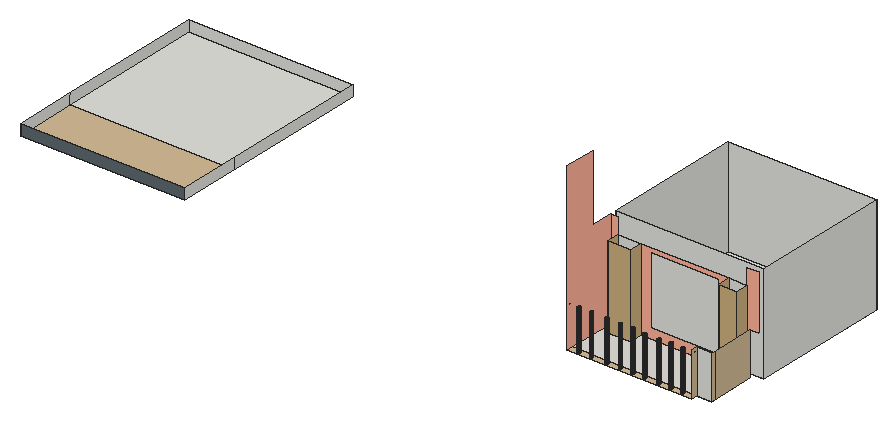
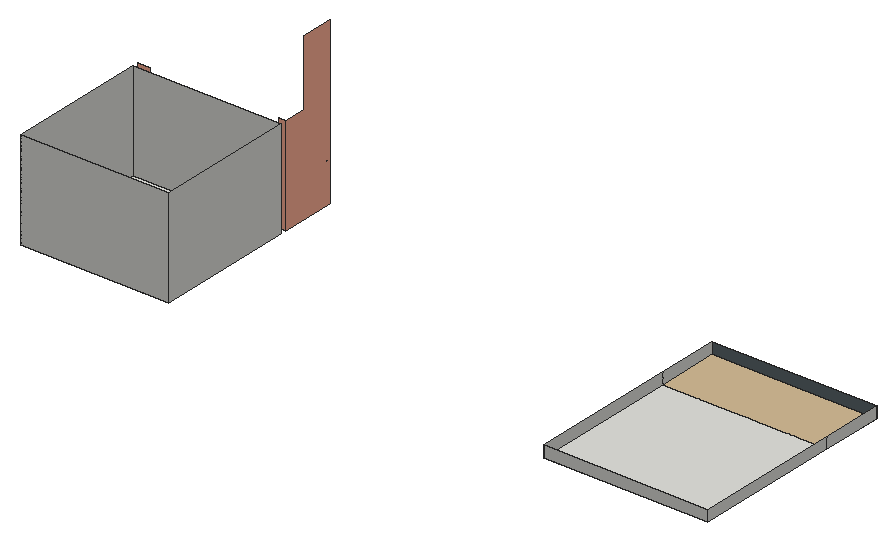
# SketchUp Ruby script. Lengths in inches.
U = 1.inch
M = Sketchup.active_model
def pt(a) = Geom::Point3d.new(a.map { |v| v * U })
def face(e, loops, mat)
  f = e.add_face(loops[0].map { |a| pt(a) })
  loops[1..].each { |l| e.add_face(l.map { |a| pt(a) }).erase! }
  f.material = f.back_material = mat if mat
  f
end
# faces: each face lists its corners as indices into pts; further lists are holes
def faces(e, pts, list, mat = nil) = list.each { |f| face(e, (f[0].is_a?(Array) ? f : [f]).map { |l| l.map { |i| pts[i] } }, mat) }
# xy, xz, yz: faces in a plane at the given z, y or x. An outline is a flat list of corners, or four numbers for a rectangle; further outlines are holes
def ring(l) = l.size == 4 ? [[l[0], l[1]], [l[2], l[1]], [l[2], l[3]], [l[0], l[3]]] : l.each_slice(2).to_a
def flat(e, list, mat, &to3) = list.each { |f| face(e, (f[0].is_a?(Array) ? f : [f]).map { |l| ring(l).map { |u, v| to3.(u, v) } }, mat) }
def xy(e, z, list, mat = nil) = flat(e, list, mat) { |x, y| [x, y, z] }
def xz(e, y, list, mat = nil) = flat(e, list, mat) { |x, z| [x, y, z] }
def yz(e, x, list, mat = nil) = flat(e, list, mat) { |y, z| [x, y, z] }
def lines(e, pts, list) = list.each { |a, b| e.add_line(pt(pts[a]), pt(pts[b])) }
# prism: a flat outline (further loops are holes) pulled along v
def prism(e, loops, v, mat = nil)
  f = face(e, loops, mat); d = Geom::Vector3d.new(v.map { |x| x * U })
  f.pushpull(f.normal.samedirection?(d) ? d.length : -d.length)
end
def box(e, o, s, mat = nil) = prism(e, [[o, [o[0] + s[0], o[1], o[2]], [o[0] + s[0], o[1] + s[1], o[2]], [o[0], o[1] + s[1], o[2]]]], [0, 0, s[2]], mat)
def at(x, y, z, deg = 0) = Geom::Transformation.translation(pt([x, y, z])) * Geom::Transformation.rotation(ORIGIN, Z_AXIS, deg.degrees)
def axes(o, x, y, z) = Geom::Transformation.new([*x, 0, *y, 0, *z, 0, *pt(o).to_a, 1])
def part(name) = M.definitions.add(name)
# library, detail: a bought-in or finely detailed component or shape, given as its bounding box
def library(name, o, s) = part(name).tap { |d| box(d.entities, o, s) }
def detail(e, o, s) = box(e.add_group.entities, o, s)
def put(e, d, t, mat = nil) = e.add_instance(d, t).tap { |i| i.material = mat if mat }
def group(e, t, mat = nil) = e.add_group.tap { |g| g.transformation = t; g.material = mat if mat }.entities
root = M.entities
M.materials.add("[Color B02]").color = [255, 178, 153]
M.materials.add("[Formica Beige]").color = [211, 187, 149]
M.materials.add("[Formica Laminate Dark]").color = [50, 53, 60]
M.materials.add("[Formica Speckled Grey]").color = [94, 105, 111]
M.materials.add("[Terrazzo Tile Accent]").color = [224, 221, 217]
M.materials.add("[Wood Floor Light]").color = [204, 176, 127]
xy(root,501,[[621.3,124.73,620.89,124.78,620.51,124.94,620.19,125.1875,619.94,125.51,619.79,125.89,619.73,126.29,619.79,126.7,619.94,127.07,620.19,127.4,620.51,127.65,620.89,127.8,621.3,127.86,621.7,127.8,622.08,127.65,622.4,127.4,622.65,127.07,622.81,126.7,622.86,126.29,622.81,125.89,622.65,125.51,622.4,125.1875,622.08,124.94,621.7,124.78],[634.92,124.73,634.52,124.78,634.14,124.94,633.82,125.1875,633.57,125.51,633.41,125.89,633.36,126.29,633.41,126.7,633.57,127.07,633.82,127.4,634.14,127.65,634.52,127.8,634.92,127.86,635.33,127.8,635.7,127.65,636.03,127.4,636.27,127.07,636.43,126.7,636.48,126.29,636.43,125.89,636.27,125.51,636.03,125.1875,635.7,124.94,635.33,124.78],[651.73,124.73,651.33,124.78,650.95,124.94,650.63,125.1875,650.38,125.51,650.22,125.89,650.17,126.29,650.22,126.7,650.38,127.07,650.63,127.4,650.95,127.65,651.33,127.8,651.73,127.86,652.14,127.8,652.51,127.65,652.84,127.4,653.09,127.07,653.24,126.7,653.3,126.29,653.24,125.89,653.09,125.51,652.84,125.1875,652.51,124.94,652.14,124.78],[666.73,124.73,666.33,124.78,665.95,124.94,665.63,125.1875,665.38,125.51,665.22,125.89,665.17,126.29,665.22,126.7,665.38,127.07,665.63,127.4,665.95,127.65,666.33,127.8,666.73,127.86,667.14,127.8,667.51,127.65,667.84,127.4,668.09,127.07,668.24,126.7,668.3,126.29,668.24,125.89,668.09,125.51,667.84,125.1875,667.51,124.94,667.14,124.78],[680.8,124.73,680.39,124.78,680.01,124.94,679.69,125.1875,679.44,125.51,679.29,125.89,679.23,126.29,679.29,126.7,679.44,127.07,679.69,127.4,680.01,127.65,680.39,127.8,680.8,127.86,681.2,127.8,681.58,127.65,681.9,127.4,682.15,127.07,682.31,126.7,682.36,126.29,682.31,125.89,682.15,125.51,681.9,125.1875,681.58,124.94,681.2,124.78],
  [693.42,124.73,693.02,124.78,692.64,124.94,692.32,125.1875,692.07,125.51,691.91,125.89,691.86,126.29,691.91,126.7,692.07,127.07,692.32,127.4,692.64,127.65,693.02,127.8,693.42,127.86,693.83,127.8,694.2,127.65,694.53,127.4,694.77,127.07,694.93,126.7,694.98,126.29,694.93,125.89,694.77,125.51,694.53,125.1875,694.2,124.94,693.83,124.78],[709.48,124.73,709.08,124.78,708.7,124.94,708.38,125.1875,708.13,125.51,707.97,125.89,707.92,126.29,707.97,126.7,708.13,127.07,708.38,127.4,708.7,127.65,709.08,127.8,709.48,127.86,709.89,127.8,710.26,127.65,710.59,127.4,710.84,127.07,710.99,126.7,711.05,126.29,710.99,125.89,710.84,125.51,710.59,125.1875,710.26,124.94,709.89,124.78],[722.42,124.73,722.02,124.78,721.64,124.94,721.32,125.1875,721.07,125.51,720.91,125.89,720.86,126.29,720.91,126.7,721.07,127.07,721.32,127.4,721.64,127.65,722.02,127.8,722.42,127.86,722.83,127.8,723.2,127.65,723.53,127.4,723.77,127.07,723.93,126.7,723.98,126.29,723.93,125.89,723.77,125.51,723.53,125.1875,723.2,124.94,722.83,124.78],[735.61,124.73,735.2,124.78,734.83,124.94,734.5,125.1875,734.26,125.51,734.1,125.89,734.05,126.29,734.1,126.7,734.26,127.07,734.5,127.4,734.83,127.65,735.2,127.8,735.61,127.86,736.01,127.8,736.39,127.65,736.71,127.4,736.96,127.07,737.12,126.7,737.17,126.29,737.12,125.89,736.96,125.51,736.71,125.1875,736.39,124.94,736.01,124.78],[619.29,168.64,644.11,182.57],
  [741.11,168.64,761.42,182.57],[611.125,189.24,774.15,344.36],[9,191.15,189.57,355.125]])
xy(root,501,[[9,122.79,189.57,191.15],[[611.125,122.79,748.22,130.07],[621.3,124.73,620.89,124.78,620.51,124.94,620.19,125.1875,619.94,125.51,619.79,125.89,619.73,126.29,619.79,126.7,619.94,127.07,620.19,127.4,620.51,127.65,620.89,127.8,621.3,127.86,621.7,127.8,622.08,127.65,622.4,127.4,622.65,127.07,622.81,126.7,622.86,126.29,622.81,125.89,622.65,125.51,622.4,125.1875,622.08,124.94,621.7,124.78],[722.42,124.73,722.02,124.78,721.64,124.94,721.32,125.1875,721.07,125.51,720.91,125.89,720.86,126.29,720.91,126.7,721.07,127.07,721.32,127.4,721.64,127.65,722.02,127.8,722.42,127.86,722.83,127.8,723.2,127.65,723.53,127.4,723.77,127.07,723.93,126.7,723.98,126.29,723.93,125.89,723.77,125.51,723.53,125.1875,723.2,124.94,722.83,124.78],[634.92,124.73,634.52,124.78,634.14,124.94,633.82,125.1875,633.57,125.51,633.41,125.89,633.36,126.29,633.41,126.7,633.57,127.07,633.82,127.4,634.14,127.65,634.52,127.8,634.92,127.86,635.33,127.8,635.7,127.65,636.03,127.4,636.27,127.07,636.43,126.7,636.48,126.29,636.43,125.89,636.27,125.51,636.03,125.1875,635.7,124.94,635.33,124.78],[709.48,124.73,709.08,124.78,708.7,124.94,708.38,125.1875,708.13,125.51,707.97,125.89,707.92,126.29,707.97,126.7,708.13,127.07,708.38,127.4,708.7,127.65,709.08,127.8,709.48,127.86,709.89,127.8,710.26,127.65,710.59,127.4,710.84,127.07,710.99,126.7,711.05,126.29,710.99,125.89,710.84,125.51,710.59,125.1875,710.26,124.94,709.89,124.78],[651.73,124.73,651.33,124.78,650.95,124.94,650.63,125.1875,650.38,125.51,650.22,125.89,650.17,126.29,650.22,126.7,650.38,127.07,650.63,127.4,650.95,127.65,651.33,127.8,651.73,127.86,652.14,127.8,652.51,127.65,652.84,127.4,653.09,127.07,653.24,126.7,653.3,126.29,653.24,125.89,653.09,125.51,652.84,125.1875,652.51,124.94,652.14,124.78],[693.42,124.73,693.02,124.78,692.64,124.94,692.32,125.1875,692.07,125.51,691.91,125.89,691.86,126.29,691.91,126.7,692.07,127.07,692.32,127.4,692.64,127.65,693.02,127.8,693.42,127.86,693.83,127.8,694.2,127.65,694.53,127.4,694.77,127.07,694.93,126.7,694.98,126.29,694.93,125.89,694.77,125.51,694.53,125.1875,694.2,124.94,693.83,124.78],[666.73,124.73,666.33,124.78,665.95,124.94,665.63,125.1875,665.38,125.51,665.22,125.89,665.17,126.29,665.22,126.7,665.38,127.07,665.63,127.4,665.95,127.65,666.33,127.8,666.73,127.86,667.14,127.8,667.51,127.65,667.84,127.4,668.09,127.07,668.24,126.7,668.3,126.29,668.24,125.89,668.09,125.51,667.84,125.1875,667.51,124.94,667.14,124.78],[680.8,124.73,680.39,124.78,680.01,124.94,679.69,125.1875,679.44,125.51,679.29,125.89,679.23,126.29,679.29,126.7,679.44,127.07,679.69,127.4,680.01,127.65,680.39,127.8,680.8,127.86,681.2,127.8,681.58,127.65,681.9,127.4,682.15,127.07,682.31,126.7,682.36,126.29,682.31,125.89,682.15,125.51,681.9,125.1875,681.58,124.94,681.2,124.78],[735.61,124.73,735.2,124.78,734.83,124.94,734.5,125.1875,734.26,125.51,734.1,125.89,734.05,126.29,734.1,126.7,734.26,127.07,734.5,127.4,734.83,127.65,735.2,127.8,735.61,127.86,736.01,127.8,736.39,127.65,736.71,127.4,736.96,127.07,737.12,126.7,737.17,126.29,737.12,125.89,736.96,125.51,736.71,125.1875,736.39,124.94,736.01,124.78]]],"[Formica Beige]")
xy(root,501,[[611.125,130.07,764.59,130.07,764.59,182.57,761.42,182.57,761.42,168.64,741.11,168.64,741.11,182.57,644.11,182.57,644.11,168.64,619.29,168.64,619.29,182.57,611.125,182.57]],"[Terrazzo Tile Accent]")
xz(root,122.79,[[9,501,189.57,513]],"[Formica Speckled Grey]")
xz(root,130.07,[[748.22,501,764.59,549]])
xz(root,168.64,[[619.29,501,644.11,591.38],[741.11,501,761.42,591.38]],"[Wood Floor Light]")
xz(root,182.57,[[619.29,501,644.11,591.38],[741.11,501,761.42,591.38]])
xz(root,182.57,[[611.125,501,619.29,609],[[644.11,501,741.11,591.38],[654.83,511.625,730.21,587]],[761.42,501,764.59,501,764.59,549,774.15,549,774.15,609,761.42,609]],"[Color B02]")
xz(root,189.24,[[611.125,501,774.15,609]])
xz(root,344.36,[[611.125,501,774.15,609]])
xz(root,355.125,[[9,501,189.57,513]])
yz(root,9,[[122.79,501,191.15,513],[191.15,501,355.125,513]])
yz(root,189.57,[[122.79,501,191.15,513],[191.15,501,355.125,513]])
yz(root,611.125,[[189.24,501,344.36,609]])
yz(root,611.125,[[[122.79,501,182.57,501,182.57,609,157.7,609,157.7,682.5,122.79,682.5],[126.51,543.63,126.14,543.68,125.79,543.82,125.49,544.05,125.26,544.35,125.12,544.69,125.07,545.07,125.12,545.4375,125.26,545.78,125.49,546.08,125.79,546.31,126.14,546.45,126.51,546.5,126.88,546.45,127.23,546.31,127.52,546.08,127.75,545.78,127.9,545.4375,127.95,545.07,127.9,544.69,127.75,544.35,127.52,544.05,127.23,543.82,126.88,543.68]]],"[Color B02]")
yz(root,619.29,[[168.64,501,182.57,591.38]],"[Wood Floor Light]")
yz(root,644.11,[[168.64,501,182.57,591.38]],"[Wood Floor Light]")
yz(root,741.11,[[168.64,501,182.57,591.38]],"[Wood Floor Light]")
yz(root,748.22,[[[122.79,501,130.07,549],[126.51,543.63,126.88,543.68,127.23,543.82,127.52,544.05,127.75,544.35,127.9,544.69,127.95,545.07,127.9,545.4375,127.75,545.78,127.52,546.08,127.23,546.31,126.88,546.45,126.51,546.5,126.14,546.45,125.79,546.31,125.49,546.08,125.26,545.78,125.12,545.4375,125.07,545.07,125.12,544.69,125.26,544.35,125.49,544.05,125.79,543.82,126.14,543.68]]],"[Formica Beige]")
yz(root,761.42,[[168.64,501,182.57,591.38]],"[Wood Floor Light]")
yz(root,764.59,[[130.07,501,133.51,549],[133.51,501,182.57,549]],"[Formica Beige]")
yz(root,774.15,[[189.24,501,344.36,609]])
p = [[620.89,124.78,501],[621.3,124.73,501],[621.3,124.73,545.4375],[620.89,124.78,545.4375],[621.7,124.78,501],[621.7,124.78,545.4375],
  [634.52,124.78,501],[634.92,124.73,501],[634.92,124.73,545.4375],[634.52,124.78,545.4375],[635.33,124.78,501],[635.33,124.78,545.4375],
  [651.33,124.78,501],[651.73,124.73,501],[651.73,124.73,545.4375],[651.33,124.78,545.4375],[652.14,124.78,501],[652.14,124.78,545.4375],
  [666.33,124.78,501],[666.73,124.73,501],[666.73,124.73,544.8125],[666.33,124.78,544.8125],[667.14,124.78,501],[667.14,124.78,544.8125],
  [680.39,124.78,501],[680.8,124.73,501],[680.8,124.73,545.78],[680.39,124.78,545.78],[681.2,124.78,501],[681.2,124.78,545.78],
  [693.02,124.78,501],[693.42,124.73,501],[693.42,124.73,544.8125],[693.02,124.78,544.8125],[693.83,124.78,501],[693.83,124.78,544.8125],
  [709.08,124.78,501],[709.48,124.73,501],[709.48,124.73,544.8125],[709.08,124.78,544.8125],[709.89,124.78,501],[709.89,124.78,544.8125],
  [722.02,124.78,501],[722.42,124.73,501],[722.42,124.73,545.78],[722.02,124.78,545.78],[722.83,124.78,501],[722.83,124.78,545.78],
  [735.2,124.78,501],[735.61,124.73,501],[735.61,124.73,545.4375],[735.2,124.78,545.4375],[736.01,124.78,501],[736.01,124.78,545.4375],
  [620.51,124.94,501],[620.51,124.94,545.4375],[622.08,124.94,501],[622.08,124.94,545.4375],[634.14,124.94,501],[634.14,124.94,545.4375],
  [635.7,124.94,501],[635.7,124.94,545.4375],[650.95,124.94,501],[650.95,124.94,545.4375],[652.51,124.94,501],[652.51,124.94,545.4375],
  [665.95,124.94,501],[665.95,124.94,544.8125],[667.51,124.94,501],[667.51,124.94,544.8125],[680.01,124.94,501],[680.01,124.94,545.78],
  [681.58,124.94,501],[681.58,124.94,545.78],[692.64,124.94,501],[692.64,124.94,544.8125],[694.2,124.94,501],[694.2,124.94,544.8125],
  [708.7,124.94,501],[708.7,124.94,544.8125],[710.26,124.94,501],[710.26,124.94,544.8125],[721.64,124.94,501],[721.64,124.94,545.78],
  [723.2,124.94,501],[723.2,124.94,545.78],[734.83,124.94,501],[734.83,124.94,545.4375],[736.39,124.94,501],[736.39,124.94,545.4375],
  [620.19,125.1875,501],[620.28,125.12,545.4375],[620.19,125.1875,545.4375],[622.4,125.1875,501],[622.4,125.1875,545.4375],[622.3125,125.12,545.4375],
  [633.82,125.1875,501],[633.91,125.12,545.4375],[633.82,125.1875,545.4375],[636.03,125.1875,501],[636.03,125.1875,545.4375],[635.9375,125.12,545.4375],
  [650.63,125.1875,501],[650.72,125.12,545.4375],[650.63,125.1875,545.4375],[652.84,125.1875,501],[652.84,125.1875,545.4375],[652.75,125.12,545.4375],
  [665.63,125.1875,501],[665.63,125.1875,544.8125],[667.84,125.1875,501],[667.84,125.1875,544.8125],[679.69,125.1875,501],[679.69,125.1875,545.78],
  [681.9,125.1875,501],[681.9,125.1875,545.78],[692.32,125.1875,501],[692.32,125.1875,544.8125],[694.53,125.1875,501],[694.53,125.1875,544.8125],
  [708.38,125.1875,501],[708.38,125.1875,544.8125],[710.59,125.1875,501],[710.59,125.1875,544.8125],[721.32,125.1875,501],[721.32,125.1875,545.78],
  [723.53,125.1875,501],[723.53,125.1875,545.78],[734.5,125.1875,501],[734.59,125.12,545.4375],[734.5,125.1875,545.4375],[736.71,125.1875,501],
  [736.71,125.1875,545.4375],[736.625,125.12,545.4375],[619.94,125.51,501],[619.94,125.51,545.4375],[622.65,125.51,501],[622.65,125.51,545.4375],
  [633.57,125.51,501],[633.57,125.51,545.4375],[636.27,125.51,501],[636.27,125.51,545.4375],[650.38,125.51,501],[650.38,125.51,545.4375],
  [653.09,125.51,501],[653.09,125.51,545.4375],[665.38,125.51,501],[665.38,125.51,544.8125],[668.09,125.51,501],[668.09,125.51,544.8125],
  [679.44,125.51,501],[679.63,125.26,545.78],[679.44,125.51,545.78],[682.15,125.51,501],[682.15,125.51,545.78],[681.96,125.26,545.78],
  [692.07,125.51,501],[692.07,125.51,544.8125],[694.77,125.51,501],[694.77,125.51,544.8125],[708.13,125.51,501],[708.13,125.51,544.8125],
  [710.84,125.51,501],[710.84,125.51,544.8125],[721.07,125.51,501],[721.26,125.26,545.78],[721.07,125.51,545.78],[723.77,125.51,501],
  [723.77,125.51,545.78],[723.58,125.26,545.78],[734.26,125.51,501],[734.26,125.51,545.4375],[736.96,125.51,501],[736.96,125.51,545.4375],
  [619.79,125.89,501],[619.79,125.89,545.4375],[622.81,125.89,501],[622.81,125.89,545.4375],[633.41,125.89,501],[633.41,125.89,545.4375],
  [636.43,125.89,501],[636.43,125.89,545.4375],[650.22,125.89,501],[650.22,125.89,545.4375],[653.24,125.89,501],[653.24,125.89,545.4375],
  [665.22,125.89,501],[665.22,125.89,544.8125],[668.24,125.89,501],[668.24,125.89,544.8125],[679.29,125.89,501],[679.29,125.89,545.78],
  [682.31,125.89,501],[682.31,125.89,545.78],[691.91,125.89,501],[691.91,125.89,544.8125],[694.93,125.89,501],[694.93,125.89,544.8125],
  [707.97,125.89,501],[707.97,125.89,544.8125],[710.99,125.89,501],[710.99,125.89,544.8125],[720.91,125.89,501],[720.91,125.89,545.78],
  [723.93,125.89,501],[723.93,125.89,545.78],[734.1,125.89,501],[734.1,125.89,545.4375],[737.12,125.89,501],[737.12,125.89,545.4375],
  [619.73,126.29,501],[619.73,126.29,545.4375],[622.86,126.29,501],[622.86,126.29,545.4375],[633.36,126.29,501],[633.36,126.29,545.4375],
  [636.48,126.29,501],[636.48,126.29,545.4375],[650.17,126.29,501],[650.17,126.29,545.4375],[653.3,126.29,501],[653.3,126.29,545.4375],
  [665.17,126.29,501],[665.17,126.29,544.8125],[668.3,126.29,501],[668.3,126.29,544.8125],[679.23,126.29,501],[679.23,126.29,545.78],
  [682.36,126.29,501],[682.36,126.29,545.78],[691.86,126.29,501],[691.86,126.29,544.8125],[694.98,126.29,501],[694.98,126.29,544.8125],
  [707.92,126.29,501],[707.92,126.29,544.8125],[711.05,126.29,501],[711.05,126.29,544.8125],[720.86,126.29,501],[720.86,126.29,545.78],
  [723.98,126.29,501],[723.98,126.29,545.78],[734.05,126.29,501],[734.05,126.29,545.4375],[737.17,126.29,501],[737.17,126.29,545.4375],
  [619.79,126.7,501],[619.79,126.7,545.4375],[622.81,126.7,501],[622.81,126.7,545.4375],[633.41,126.7,501],[633.41,126.7,545.4375],
  [636.43,126.7,501],[636.43,126.7,545.4375],[650.22,126.7,501],[650.22,126.7,545.4375],[653.24,126.7,501],[653.24,126.7,545.4375],
  [665.22,126.7,501],[665.22,126.7,544.8125],[668.24,126.7,501],[668.24,126.7,544.8125],[679.29,126.7,501],[679.29,126.7,545.78],
  [682.31,126.7,501],[682.31,126.7,545.78],[691.91,126.7,501],[691.91,126.7,544.8125],[694.93,126.7,501],[694.93,126.7,544.8125],
  [707.97,126.7,501],[707.97,126.7,544.8125],[710.99,126.7,501],[710.99,126.7,544.8125],[720.91,126.7,501],[720.91,126.7,545.78],
  [723.93,126.7,501],[723.93,126.7,545.78],[734.1,126.7,501],[734.1,126.7,545.4375],[737.12,126.7,501],[737.12,126.7,545.4375],
  [619.94,127.07,501],[619.94,127.07,545.4375],[622.65,127.07,501],[622.65,127.07,545.4375],[633.57,127.07,501],[633.57,127.07,545.4375],
  [636.27,127.07,501],[636.27,127.07,545.4375],[650.38,127.07,501],[650.38,127.07,545.4375],[653.09,127.07,501],[653.09,127.07,545.4375],
  [665.38,127.07,501],[665.38,127.07,544.8125],[668.09,127.07,501],[668.09,127.07,544.8125],[679.44,127.07,501],[679.44,127.07,545.78],
  [682.15,127.07,501],[682.15,127.07,545.78],[692.07,127.07,501],[692.07,127.07,544.8125],[694.77,127.07,501],[694.77,127.07,544.8125],
  [708.13,127.07,501],[708.13,127.07,544.8125],[710.84,127.07,501],[710.84,127.07,544.8125],[721.07,127.07,501],[721.07,127.07,545.78],
  [723.77,127.07,501],[723.77,127.07,545.78],[734.26,127.07,501],[734.26,127.07,545.4375],[736.96,127.07,501],[736.96,127.07,545.4375],
  [620.19,127.4,501],[620.19,127.4,545.4375],[622.4,127.4,501],[622.4,127.4,545.4375],[633.82,127.4,501],[633.82,127.4,545.4375],
  [636.03,127.4,501],[636.03,127.4,545.4375],[650.63,127.4,501],[650.63,127.4,545.4375],[652.84,127.4,501],[652.84,127.4,545.4375],
  [665.63,127.4,501],[665.63,127.4,544.8125],[667.84,127.4,501],[667.84,127.4,544.8125],[679.69,127.4,501],[679.69,127.4,545.78],
  [681.9,127.4,501],[681.9,127.4,545.78],[692.32,127.4,501],[692.32,127.4,544.8125],[694.53,127.4,501],[694.53,127.4,544.8125],
  [708.38,127.4,501],[708.38,127.4,544.8125],[710.59,127.4,501],[710.59,127.4,544.8125],[721.32,127.4,501],[721.32,127.4,545.78],
  [723.53,127.4,501],[723.53,127.4,545.78],[734.5,127.4,501],[734.5,127.4,545.4375],[736.71,127.4,501],[736.71,127.4,545.4375],
  [620.51,127.65,501],[620.51,127.65,545.4375],[622.08,127.65,501],[622.08,127.65,545.4375],[634.14,127.65,501],[634.14,127.65,545.4375],
  [635.7,127.65,501],[635.7,127.65,545.4375],[650.95,127.65,501],[650.95,127.65,545.4375],[652.51,127.65,501],[652.51,127.65,545.4375],
  [665.95,127.65,501],[665.95,127.65,544.8125],[667.51,127.65,501],[667.51,127.65,544.8125],[680.01,127.65,501],[680.01,127.65,545.78],
  [681.58,127.65,501],[681.58,127.65,545.78],[692.64,127.65,501],[692.64,127.65,544.8125],[694.2,127.65,501],[694.2,127.65,544.8125],
  [708.7,127.65,501],[708.7,127.65,544.8125],[710.26,127.65,501],[710.26,127.65,544.8125],[721.64,127.65,501],[721.64,127.65,545.78],
  [723.2,127.65,501],[723.2,127.65,545.78],[734.83,127.65,501],[734.83,127.65,545.4375],[736.39,127.65,501],[736.39,127.65,545.4375],
  [620.89,127.8,501],[620.89,127.8,545.4375],[621.7,127.8,501],[621.7,127.8,545.4375],[634.52,127.8,501],[634.52,127.8,545.4375],
  [635.33,127.8,501],[635.33,127.8,545.4375],[651.33,127.8,501],[651.33,127.8,545.4375],[652.14,127.8,501],[652.14,127.8,545.4375],
  [666.33,127.8,501],[666.33,127.8,544.8125],[667.14,127.8,501],[667.14,127.8,544.8125],[680.39,127.8,501],[680.27,127.75,545.78],
  [680.39,127.8,545.78],[681.2,127.8,501],[681.2,127.8,545.78],[681.32,127.75,545.78],[693.02,127.8,501],[693.02,127.8,544.8125],
  [693.83,127.8,501],[693.83,127.8,544.8125],[709.08,127.8,501],[709.08,127.8,544.8125],[709.89,127.8,501],[709.89,127.8,544.8125],
  [722.02,127.8,501],[721.9,127.75,545.78],[722.02,127.8,545.78],[722.83,127.8,501],[722.83,127.8,545.78],[722.95,127.75,545.78],
  [735.2,127.8,501],[735.2,127.8,545.4375],[736.01,127.8,501],[736.01,127.8,545.4375],[621.3,127.86,501],[621.3,127.86,545.4375],
  [634.92,127.86,501],[634.92,127.86,545.4375],[651.73,127.86,501],[651.73,127.86,545.4375],[666.73,127.86,501],[666.73,127.86,544.8125],
  [680.8,127.86,501],[680.8,127.86,545.78],[693.42,127.86,501],[693.42,127.86,544.8125],[709.48,127.86,501],[709.48,127.86,544.8125],
  [722.42,127.86,501],[722.42,127.86,545.78],[735.61,127.86,501],[735.61,127.86,545.4375]]
faces(root,p,[[0,1,2,3],[1,4,5,2],[6,7,8,9],[7,10,11,8],[12,13,14,15],[13,16,17,14],[18,19,20,21],[19,22,23,20],
  [24,25,26,27],[25,28,29,26],[30,31,32,33],[31,34,35,32],[36,37,38,39],[37,40,41,38],[42,43,44,45],[43,46,47,44],
  [48,49,50,51],[49,52,53,50],[54,0,3,55],[4,56,57,5],[58,6,9,59],[10,60,61,11],[62,12,15,63],[16,64,65,17],
  [66,18,21,67],[22,68,69,23],[70,24,27,71],[28,72,73,29],[74,30,33,75],[34,76,77,35],[78,36,39,79],[40,80,81,41],
  [82,42,45,83],[46,84,85,47],[86,48,51,87],[52,88,89,53],[90,54,55,91,92],[56,93,94,95,57],[96,58,59,97,98],[60,99,100,101,61],
  [102,62,63,103,104],[64,105,106,107,65],[108,66,67,109],[68,110,111,69],[112,70,71,113],[72,114,115,73],[116,74,75,117],[76,118,119,77],
  [120,78,79,121],[80,122,123,81],[124,82,83,125],[84,126,127,85],[128,86,87,129,130],[88,131,132,133,89],[134,90,92,135],[93,136,137,94],
  [138,96,98,139],[99,140,141,100],[142,102,104,143],[105,144,145,106],[146,108,109,147],[110,148,149,111],[150,112,113,151,152],[114,153,154,155,115],
  [156,116,117,157],[118,158,159,119],[160,120,121,161],[122,162,163,123],[164,124,125,165,166],[126,167,168,169,127],[170,128,130,171],[131,172,173,132],
  [174,134,135,175],[136,176,177,137],[178,138,139,179],[140,180,181,141],[182,142,143,183],[144,184,185,145],[186,146,147,187],[148,188,189,149],
  [190,150,152,191],[153,192,193,154],[194,156,157,195],[158,196,197,159],[198,160,161,199],[162,200,201,163],[202,164,166,203],[167,204,205,168],
  [206,170,171,207],[172,208,209,173],[210,174,175,211],[176,212,213,177],[214,178,179,215],[180,216,217,181],[218,182,183,219],[184,220,221,185],
  [222,186,187,223],[188,224,225,189],[226,190,191,227],[192,228,229,193],[230,194,195,231],[196,232,233,197],[234,198,199,235],[200,236,237,201],
  [238,202,203,239],[204,240,241,205],[242,206,207,243],[208,244,245,209],[246,210,211,247],[212,248,249,213],[250,214,215,251],[216,252,253,217],
  [254,218,219,255],[220,256,257,221],[258,222,223,259],[224,260,261,225],[262,226,227,263],[228,264,265,229],[266,230,231,267],[232,268,269,233],
  [270,234,235,271],[236,272,273,237],[274,238,239,275],[240,276,277,241],[278,242,243,279],[244,280,281,245],[282,246,247,283],[248,284,285,249],
  [286,250,251,287],[252,288,289,253],[290,254,255,291],[256,292,293,257],[294,258,259,295],[260,296,297,261],[298,262,263,299],[264,300,301,265],
  [302,266,267,303],[268,304,305,269],[306,270,271,307],[272,308,309,273],[310,274,275,311],[276,312,313,277],[314,278,279,315],[280,316,317,281],
  [318,282,283,319],[284,320,321,285],[322,286,287,323],[288,324,325,289],[326,290,291,327],[292,328,329,293],[330,294,295,331],[296,332,333,297],
  [334,298,299,335],[300,336,337,301],[338,302,303,339],[304,340,341,305],[342,306,307,343],[308,344,345,309],[346,310,311,347],[312,348,349,313],
  [350,314,315,351],[316,352,353,317],[354,318,319,355],[320,356,357,321],[358,322,323,359],[324,360,361,325],[362,326,327,363],[328,364,365,329],
  [366,330,331,367],[332,368,369,333],[370,334,335,371],[336,372,373,337],[374,338,339,375],[340,376,377,341],[378,342,343,379],[344,380,381,345],
  [382,346,347,383],[348,384,385,349],[386,350,351,387],[352,388,389,353],[390,354,355,391],[356,392,393,357],[394,358,359,395],[360,396,397,361],
  [398,362,363,399],[364,400,401,365],[402,366,367,403],[368,404,405,369],[406,370,371,407,408],[372,409,410,411,373],[412,374,375,413],[376,414,415,377],
  [416,378,379,417],[380,418,419,381],[420,382,383,421,422],[384,423,424,425,385],[426,386,387,427],[388,428,429,389],[430,390,391,431],[392,430,431,393],
  [432,394,395,433],[396,432,433,397],[434,398,399,435],[400,434,435,401],[436,402,403,437],[404,436,437,405],[438,406,408,439],[409,438,439,410],
  [440,412,413,441],[414,440,441,415],[442,416,417,443],[418,442,443,419],[444,420,422,445],[423,444,445,424],[446,426,427,447],[428,446,447,429]],"[Formica Laminate Dark]")
